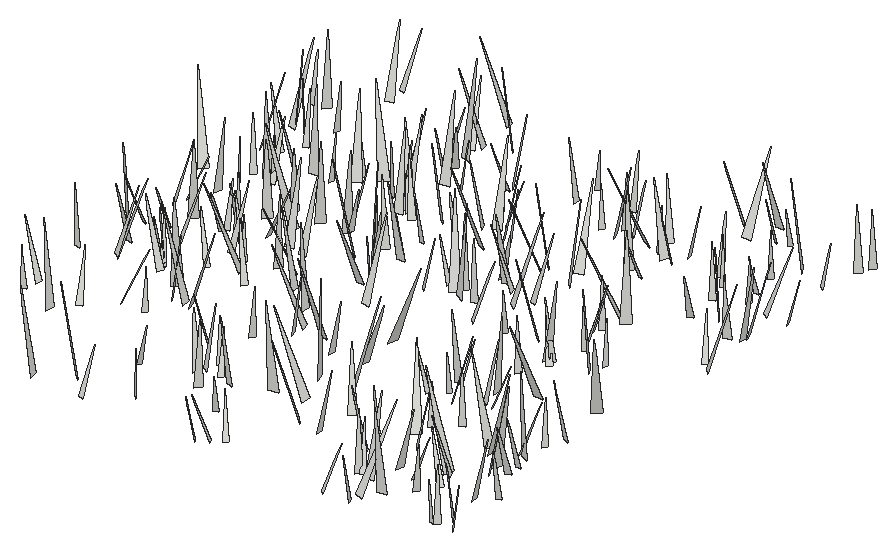
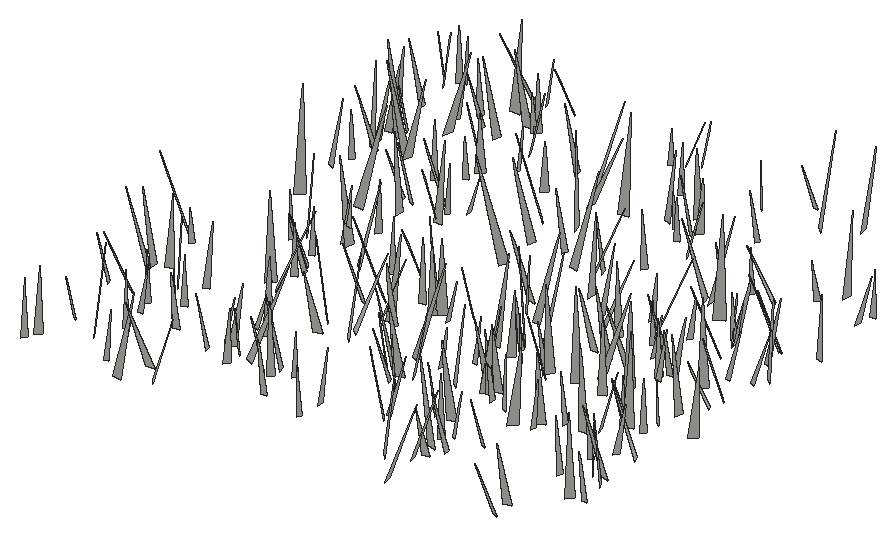
# SketchUp Ruby script. Lengths in inches.
U = 1.inch
M = Sketchup.active_model
def pt(a) = Geom::Point3d.new(a.map { |v| v * U })
def face(e, loops, mat)
  f = e.add_face(loops[0].map { |a| pt(a) })
  loops[1..].each { |l| e.add_face(l.map { |a| pt(a) }).erase! }
  f.material = f.back_material = mat if mat
  f
end
# faces: each face lists its corners as indices into pts; further lists are holes
def faces(e, pts, list, mat = nil) = list.each { |f| face(e, (f[0].is_a?(Array) ? f : [f]).map { |l| l.map { |i| pts[i] } }, mat) }
# xy, xz, yz: faces in a plane at the given z, y or x. An outline is a flat list of corners, or four numbers for a rectangle; further outlines are holes
def ring(l) = l.size == 4 ? [[l[0], l[1]], [l[2], l[1]], [l[2], l[3]], [l[0], l[3]]] : l.each_slice(2).to_a
def flat(e, list, mat, &to3) = list.each { |f| face(e, (f[0].is_a?(Array) ? f : [f]).map { |l| ring(l).map { |u, v| to3.(u, v) } }, mat) }
def xy(e, z, list, mat = nil) = flat(e, list, mat) { |x, y| [x, y, z] }
def xz(e, y, list, mat = nil) = flat(e, list, mat) { |x, z| [x, y, z] }
def yz(e, x, list, mat = nil) = flat(e, list, mat) { |y, z| [x, y, z] }
def lines(e, pts, list) = list.each { |a, b| e.add_line(pt(pts[a]), pt(pts[b])) }
# prism: a flat outline (further loops are holes) pulled along v
def prism(e, loops, v, mat = nil)
  f = face(e, loops, mat); d = Geom::Vector3d.new(v.map { |x| x * U })
  f.pushpull(f.normal.samedirection?(d) ? d.length : -d.length)
end
def box(e, o, s, mat = nil) = prism(e, [[o, [o[0] + s[0], o[1], o[2]], [o[0] + s[0], o[1] + s[1], o[2]], [o[0], o[1] + s[1], o[2]]]], [0, 0, s[2]], mat)
def at(x, y, z, deg = 0) = Geom::Transformation.translation(pt([x, y, z])) * Geom::Transformation.rotation(ORIGIN, Z_AXIS, deg.degrees)
def axes(o, x, y, z) = Geom::Transformation.new([*x, 0, *y, 0, *z, 0, *pt(o).to_a, 1])
def part(name) = M.definitions.add(name)
# library, detail: a bought-in or finely detailed component or shape, given as its bounding box
def library(name, o, s) = part(name).tap { |d| box(d.entities, o, s) }
def detail(e, o, s) = box(e.add_group.entities, o, s)
def put(e, d, t, mat = nil) = e.add_instance(d, t).tap { |i| i.material = mat if mat }
def group(e, t, mat = nil) = e.add_group.tap { |g| g.transformation = t; g.material = mat if mat }.entities
root = M.entities
c1 = part("fur_instance\#9")
p = [[0.8125,0,1.79],[0.67,-0.02,1.48],[0,-0.11,0],[0,0.11,0]]
faces(c1.entities,p,[[0,1,2,3]])
put(root,c1,axes([503.7,262.17,-21.66],[2.36967,1.89121,2.13493],[2.35412,-2.86396,-0.07595],[-1.61018,-1.40392,3.03088]))
put(root,c1,axes([532.14,262.03,-21.66],[-3.28529,-1.60429,1.12724],[-1.66632,3.44368,0.04462],[1.03333,0.45264,3.6558]))
put(root,c1,axes([473.92,262.57,-21.66],[-6.8866,-1.44069,2.04712],[-1.4724,7.17733,0.09795],[2.02444,0.3193,7.035]))
put(root,c1,axes([505.68,263.29,-21.66],[-3.47734,-1.80435,0.22841],[-1.8088,3.48242,-0.02761],[0.19,0.12974,3.9175]))
put(root,c1,axes([527.41,261.63,-21.66],[2.54826,3.20038,0.28055],[3.20908,-2.5526,-0.02947],[-0.15164,-0.23787,4.09087]))
put(root,c1,axes([483.3,261.68,-21.66],[0.89706,4.01856,0.51185],[4.05094,-0.89322,-0.08685],[-0.02607,-0.51851,4.11655]))
put(root,c1,axes([545.09,264.49,-21.66],[-0.48209,-3.49328,1.24378],[-3.69826,0.54426,0.09516],[0.26993,1.21786,3.5251]))
put(root,c1,axes([546.02,264.64,-21.66],[-2.69115,3.5868,1.84623],[3.86426,2.92918,-0.05799],[1.15809,-1.43902,4.48375]))
put(root,c1,axes([548.86,264.65,-21.66],[-2.22453,-2.28888,1.93607],[-2.6411,2.63697,0.08289],[1.41842,1.32035,3.19071]))
put(root,c1,axes([479,266.04,-21.66],[-5.20637,-5.83633,2.28098],[-6.06397,5.44004,0.07832],[1.57922,1.64775,7.82067]))
put(root,c1,axes([507.56,264.51,-21.66],[-2.46678,3.0111,0.36551],[3.02886,2.4705,0.08915],[0.1623,-0.33942,3.8915]))
put(root,c1,axes([534.27,266.7,-21.66],[0.04247,-7.07988,2.41623],[-7.48051,-0.06275,-0.05238],[-0.06984,2.41579,7.07981]))
put(root,c1,axes([489.21,266.67,-21.66],[-2.0645,-2.99831,1.70133],[-3.28642,2.31061,0.08412],[1.04107,1.34824,3.63936]))
put(root,c1,axes([547.11,267.03,-21.66],[-3.81411,-2.18756,1.38745],[-2.30966,3.98998,-0.05835],[1.17299,0.74331,4.39652]))
put(root,c1,axes([532.3125,263.92,-21.66],[2.76635,7.35948,0.05567],[7.35952,-2.76581,-0.07342],[0.04914,-0.07794,7.86188]))
put(root,c1,axes([500.875,270.59,-21.66],[2.15592,-3.18911,0.31319],[-3.19535,-2.16794,-0.07942],[-0.24138,0.21478,3.84865]))
put(root,c1,axes([528.03,269.25,-21.66],[-3.99726,2.72851,1.81883],[2.89094,4.28575,-0.07581],[1.5477,-0.9584,4.83912]))
put(root,c1,axes([537.71,270.27,-21.66],[-2.80028,2.24736,2.49663],[2.73085,3.4158,-0.01176],[1.95607,-1.55147,3.59055]))
put(root,c1,axes([530.31,268.78,-21.66],[0.3651,6.79595,1.75212],[7.01816,-0.34958,-0.10649],[0.01583,-1.75528,6.80491]))
put(root,c1,axes([528.58,269.49,-21.66],[-2.41477,3.3901,0.55663],[3.41153,2.44646,-0.10002],[0.40504,-0.3947,4.161]))
put(root,c1,axes([535.15,272.91,-21.66],[4.26673,-0.51352,0.23406],[-0.5171,-4.27238,0.05285],[-0.22604,0.08052,4.29719]))
put(root,c1,axes([531.66,274.01,-21.66],[5.79925,-1.98106,0.58125],[-1.98372,-5.82701,-0.06806],[-0.57211,0.1232,6.12791]))
put(root,c1,axes([545.76,273.52,-21.66],[5.31059,0.52385,1.16283],[0.52648,-5.43598,0.04446],[-1.16164,-0.06886,5.33618]))
put(root,c1,axes([483.73,274.41,-21.66],[3.66443,-1.25509,0.51627],[-1.25966,-3.69872,-0.05095],[-0.50503,0.11865,3.87307]))
put(root,c1,axes([539.72,273.26,-21.66],[-3.84574,2.31871,0.01808],[2.31862,3.84577,-0.02193],[0.02681,0.00945,4.49062]))
put(root,c1,axes([494.51,274.5,-21.66],[4.30224,-3.16543,2.15858],[-3.43037,-4.62804,0.05027],[-1.70646,1.32286,5.34104]))
put(root,c1,axes([511.87,275.81,-21.66],[-4.79453,-5.10071,1.01007],[-5.15614,4.84133,-0.02673],[0.67211,0.75447,7.00029]))
put(root,c1,axes([524.97,274.87,-21.66],[-4.98874,-1.77944,1.14235],[-1.81158,5.1064,0.04294],[1.09068,0.3424,5.29642]))
put(root,c1,axes([548.35,275.79,-21.66],[1.07632,-4.38935,0.89904],[-4.4763,-1.09335,0.02097],[-0.19334,0.87825,4.51934]))
put(root,c1,axes([516.25,274.92,-21.66],[5.41159,0.09186,1.28906],[0.07062,-5.56242,0.09991],[-1.29039,0.08081,5.41145]))
put(root,c1,axes([538.75,276.86,-21.66],[-4.66141,-1.64687,0.68606],[-1.65466,4.70851,0.06011],[0.66704,0.1713,4.94341]))
put(root,c1,axes([497.46,277.85,-21.66],[-1.75963,-5.21212,1.71135],[-5.46295,1.82898,-0.04671],[0.50104,1.63703,5.50093]))
put(root,c1,axes([537.97,277.33,-21.66],[-8.02945,1.44749,0.94959],[1.4539,8.08421,-0.0293],[0.93976,-0.13944,8.15883]))
put(root,c1,axes([491.58,277.75,-21.66],[-4.02288,2.74208,1.38872],[2.85785,4.17888,0.02734],[1.13147,-0.80565,4.86845]))
put(root,c1,axes([463.69,279.07,-21.66],[-6.94561,0.7265,2.56424],[0.79665,7.39636,0.06233],[2.54332,-0.33278,6.98322]))
put(root,c1,axes([503.6,280.3,-21.66],[1.30407,-7.61557,2.3618],[-7.95747,-1.39423,-0.10194],[-0.50366,2.30972,7.72574]))
put(root,c1,axes([495.13,278.84,-21.66],[-1.61358,3.38665,0.61033],[3.4322,1.63258,0.01498],[0.24881,-0.55751,3.75138]))
put(root,c1,axes([523.21,279.71,-21.66],[-3.75742,-0.36081,1.22113],[-0.40687,3.94545,-0.08619],[1.20657,0.20686,3.77372]))
put(root,c1,axes([492.12,279.05,-21.66],[2.52877,4.50107,1.40807],[4.66336,-2.62485,0.01569],[-0.70386,-1.21962,5.16276]))
put(root,c1,axes([544.91,282.3125,-21.66],[1.17594,-4.92519,0.34785],[-4.93492,-1.18388,-0.07952],[-0.1583,0.31979,5.06301]))
put(root,c1,axes([542.87,280.57,-21.66],[3.30994,1.56111,0.94089],[1.62723,-3.40964,-0.0672],[-0.82125,-0.46405,3.659]))
put(root,c1,axes([529.89,280.22,-21.66],[3.54809,3.00738,1.07129],[3.07779,-3.64774,0.04651],[-0.84804,-0.65624,4.65093]))
put(root,c1,axes([457.1,281.34,-21.66],[1.04159,-3.44564,1.2731],[-3.64709,-1.12789,-0.06873],[-0.4381,1.19732,3.59897]))
put(root,c1,axes([508.86,281.11,-21.66],[-7.40149,0.22253,0.007],[0.22253,7.40149,0.00759],[0.00677,-0.0078,7.40483]))
put(root,c1,axes([492.89,281.5,-21.66],[1.88047,-2.78184,1.95652],[-3.20631,-2.19563,-0.04014],[-1.13412,1.59479,3.35756]))
put(root,c1,axes([542.47,282.83,-21.66],[7.05562,-2.47543,1.6862],[-2.53392,-7.23407,-0.01726],[-1.59697,0.54154,7.47725]))
put(root,c1,axes([516.67,281.93,-21.66],[-3.66348,3.88372,0.60062],[3.90017,3.69385,-0.09601],[0.48235,-0.37054,5.33808]))
put(root,c1,axes([488.92,284.06,-21.66],[-3.66395,-2.75565,0.79106],[-2.79858,3.7164,-0.01609],[0.62239,0.48852,4.58453]))
put(root,c1,axes([544.86,284.65,-21.66],[-0.84306,-4.44176,0.86686],[-4.52258,0.85891,0.00263],[0.16427,0.85115,4.52106]))
put(root,c1,axes([466.31,282.45,-21.66],[-1.50833,4.20798,0.27956],[4.21722,1.50618,0.08227],[0.01672,-0.29093,4.46939]))
put(root,c1,axes([457.63,284.17,-21.66],[-4.98087,1.16288,0.32288],[1.15979,4.99131,-0.08543],[0.33384,0.00996,5.1141]))
put(root,c1,axes([527.28,283.33,-21.66],[-4.42637,5.44798,0.10976],[5.44745,4.42761,-0.08267],[0.13338,-0.03304,7.019]))
put(root,c1,axes([539.19,285.53,-21.66],[7.16515,0.1083,1.44204],[0.09788,-7.3087,0.06254],[-1.44279,0.042,7.1657]))
put(root,c1,axes([527.66,286.15,-21.66],[1.56835,-2.82264,1.69633],[-3.20586,-1.73838,0.07137],[-0.75322,1.52161,3.2283]))
put(root,c1,axes([474.875,286.87,-21.66],[-2.3678,2.48019,1.72309],[2.76192,2.66404,-0.03926],[1.22155,-1.2159,3.42875]))
put(root,c1,axes([537.98,286.61,-21.66],[-7.39383,1.79038,1.19471],[1.82356,7.48136,0.07416],[1.14343,-0.35412,7.60715]))
put(root,c1,axes([543.77,287.375,-21.66],[2.87262,5.81566,3.24646],[6.49078,-3.23727,0.05584],[-1.49368,-2.88298,6.48619]))
put(root,c1,axes([506.33,287.46,-21.66],[7.01213,2.59998,3.36264],[2.81322,-7.70163,0.08845],[-3.18638,-1.07803,7.47811]))
put(root,c1,axes([470.45,287.08,-21.66],[4.47916,2.33614,0.04477],[2.33654,-4.47877,-0.05982],[-0.01203,-0.07375,5.05142]))
put(root,c1,axes([542.66,287.96,-21.66],[5.19271,0.37939,0.34653],[0.38191,-5.20401,-0.02543],[-0.34375,-0.05067,5.20649]))
put(root,c1,axes([530.99,289.25,-21.66],[1.68942,-4.24341,1.91691],[-4.60334,-1.82876,0.00876],[-0.70022,1.78447,4.56734]))
put(root,c1,axes([511.6,288.69,-21.66],[5.53821,4.98185,1.27941],[5.04776,-5.62536,0.05401],[-0.98782,-0.81487,7.449]))
put(root,c1,axes([491.43,290.72,-21.66],[3.58428,-2.61771,1.24135],[-2.70899,-3.7283,-0.04015],[-1.02701,0.69843,4.43823]))
put(root,c1,axes([544.11,291.72,-21.66],[-2.72992,2.63061,1.69887],[2.87463,2.99911,-0.02472],[1.24209,-1.1593,3.79104]))
put(root,c1,axes([477.83,292.48,-21.66],[-7.83982,-0.95667,1.33619],[-0.96404,7.9519,0.03699],[1.33088,0.12461,7.89789]))
put(root,c1,axes([475.53,292.26,-21.66],[4.582,2.26461,1.64468],[2.3704,-4.81752,0.02956],[-1.48816,-0.70087,5.111]))
put(root,c1,axes([478.9,292.19,-21.66],[6.34041,1.92452,0.88463],[1.94009,-6.39712,0.01179],[-0.84995,-0.24555,6.62604]))
put(root,c1,axes([521.17,293.61,-21.66],[-3.91396,0.19988,0.40503],[0.19284,3.93443,-0.07818],[0.40843,0.05784,3.91828]))
put(root,c1,axes([503.17,294.04,-21.66],[4.73571,-1.08461,0.9225],[-1.0987,-4.82145,-0.02851],[-0.90568,0.17765,4.85824]))
put(root,c1,axes([508.71,294.81,-21.66],[6.16535,-1.94029,0.16764],[-1.94054,-6.16752,-0.01601],[-0.16472,0.03505,6.46343]))
put(root,c1,axes([545.17,295.05,-21.66],[-1.95958,-4.83915,1.26512],[-4.97855,2.01787,0.00704],[0.48156,1.1699,5.22085]))
put(root,c1,axes([473.6875,295.65,-21.66],[3.80262,-6.94068,2.14426],[-7.19034,-3.9408,-0.00453],[-1.0344,1.87826,7.9141]))
put(root,c1,axes([525.47,293.91,-21.66],[4.69542,3.0157,0.91715],[3.05189,-4.76105,0.03053],[-0.78841,-0.46959,5.58037]))
put(root,c1,axes([499.41,296.93,-21.66],[-2.16653,-7.31637,0.90738],[-7.36569,2.18851,0.05952],[0.3151,0.85299,7.63018]))
put(root,c1,axes([523.5,295.61,-21.66],[1.81522,-3.21568,0.8696],[-3.29805,-1.87418,-0.04607],[-0.46866,0.73395,3.69235]))
put(root,c1,axes([495.33,295.16,-21.66],[4.4988,1.24272,1.44893],[1.33102,-4.70119,-0.10058],[-1.36826,-0.48722,4.6662]))
put(root,c1,axes([455.36,295.72,-21.66],[1.09401,4.63876,2.44173],[5.21296,-1.22556,-0.00737],[-0.55243,-2.37843,4.76601]))
put(root,c1,axes([531.0625,296.09,-21.66],[3.86213,1.08614,0.2172],[1.09096,-3.86634,-0.0646],[-0.19154,-0.12107,4.01143]))
put(root,c1,axes([495.47,297.57,-21.66],[-6.50715,-2.26194,0.29712],[-2.26712,6.51165,-0.07913],[0.25462,0.17236,6.88863]))
put(root,c1,axes([529.4375,296.45,-21.66],[2.64561,4.33348,1.24236],[4.47199,-2.70465,-0.08904],[-0.56902,-1.10798,5.07645]))
put(root,c1,axes([522.83,298.63,-21.66],[0.27233,-6.25887,1.87066],[-6.53155,-0.29195,-0.02597],[-0.1084,1.8677,6.26474]))
put(root,c1,axes([469.08,297.55,-21.66],[-5.48361,2.04542,0.49712],[2.0602,5.49974,0.09665],[0.43181,-0.2646,5.85187]))
put(root,c1,axes([524,297.5625,-21.66],[2.95956,2.83712,0.75066],[2.89518,-2.997,-0.08741],[-0.48027,-0.58351,4.09885]))
put(root,c1,axes([461.68,297.09,-21.66],[4.96936,4.425,0.65774],[4.44372,-4.99597,0.03757],[-0.51632,-0.4092,6.65385]))
put(root,c1,axes([461.31,297.24,-21.66],[3.13584,4.70476,0.63652],[4.72939,-3.16238,0.0748],[-0.41563,-0.48786,5.65355]))
put(root,c1,axes([534.39,302.33,-21.66],[-0.28609,-7.90952,0.17476],[-7.91116,0.28452,-0.07401],[-0.06767,0.17732,7.91434]))
put(root,c1,axes([468.52,298.81,-21.66],[-1.71851,4.03919,1.0736],[4.16688,1.74577,0.10182],[0.32374,-1.02868,4.3884]))
put(root,c1,axes([467.48,299.8,-21.66],[-3.40834,-0.81843,0.94444],[-0.85751,3.5273,-0.03792],[0.90911,0.25869,3.50503]))
put(root,c1,axes([528.77,299.88,-21.66],[6.1687,-0.67373,2.21616],[-0.70194,-6.55164,-0.0379],[-2.20738,0.2006,6.20527]))
put(root,c1,axes([467.7,300.24,-21.66],[-3.21218,-2.63282,1.4726],[-2.81239,3.39173,-0.07071],[1.09119,0.99138,4.15269]))
put(root,c1,axes([460.17,301.5625,-21.66],[-1.26664,-5.03308,1.07763],[-5.14261,1.28411,-0.04714],[0.2163,1.05675,5.1898]))
put(root,c1,axes([507.95,302.06,-21.66],[8.10386,-2.02713,0.06413],[-2.02706,-8.10412,-0.01624],[-0.06615,-0.00019,8.35354]))
put(root,c1,axes([492.31,301.76,-21.66],[-6.58404,0.20466,2.39247],[0.20033,7.00521,-0.04793],[2.39284,-0.02336,6.58705]))
put(root,c1,axes([543.59,304.23,-21.66],[4.25947,-6.86655,0.67935],[-6.89421,-4.26807,0.08653],[-0.2843,0.62304,8.07992]))
put(root,c1,axes([481,301.82,-21.66],[-3.95377,2.90545,0.68572],[2.92437,3.99824,-0.07937],[0.59996,-0.34142,4.90588]))
put(root,c1,axes([473.61,302.51,-21.66],[-3.58743,2.64736,0.43412],[2.66538,3.59954,0.07504],[0.30449,-0.3184,4.45786]))
put(root,c1,axes([477.97,304.68,-21.66],[-6.75441,-2.93713,0.31923],[-2.94167,6.75982,-0.04619],[0.27431,0.1697,7.36523]))
put(root,c1,axes([457.1875,305.06,-21.66],[-4.34525,-4.69158,2.51984],[-5.05188,4.66036,-0.03462],[1.68493,1.87398,6.3946]))
put(root,c1,axes([487.51,305.26,-21.66],[-6.3571,-0.05635,1.63328],[-0.03082,6.56286,0.10646],[1.63396,-0.09544,6.35645]))
put(root,c1,axes([467.11,303.86,-21.66],[4.12664,4.96749,0.53315],[4.97839,-4.14664,0.10195],[-0.41933,-0.34468,6.45715]))
put(root,c1,axes([458.4375,307.16,-21.66],[-1.93771,-4.14246,0.35212],[-4.15628,1.93921,-0.05843],[0.0961,0.34375,4.57288]))
put(root,c1,axes([527.59,306.21,-21.66],[3.42061,-2.16163,2.16053],[-2.46149,-3.8706,0.02453],[-1.81151,1.17767,4.04631]))
put(root,c1,axes([461.96,308.34,-21.66],[-0.71572,-3.67555,0.46048],[-3.70429,0.70984,-0.09154],[-0.00255,0.46948,3.74347]))
put(root,c1,axes([476.59,307.19,-21.66],[-1.48065,3.15767,1.46809],[3.42197,1.61497,-0.02236],[0.64523,-1.31889,3.48751]))
put(root,c1,axes([484.46,309.35,-21.66],[-3.64802,-5.0358,0.07825],[-5.03596,3.64854,0.02575],[0.06676,0.04827,6.21825]))
put(root,c1,axes([481.78,308.7,-21.66],[5.0258,-2.8928,2.35137],[-3.11716,-5.42578,-0.01254],[-2.04464,1.16127,5.79886]))
put(root,c1,axes([473.82,307.8125,-21.66],[1.01663,5.56132,0.68679],[5.60282,-1.02017,-0.03274],[-0.09106,-0.68151,5.65338]))
put(root,c1,axes([493.64,312.56,-21.66],[-0.44109,-6.89492,0.21564],[-6.89758,0.44393,0.08524],[0.09888,0.20974,6.90849]))
put(root,c1,axes([498.125,308.09,-21.66],[1.00933,7.00307,0.82634],[7.04916,-1.02422,0.06983],[-0.18746,-0.80782,7.07509]))
put(root,c1,axes([468.7,312.03,-21.66],[0.77798,-4.23548,0.16889],[-4.23878,-0.77834,0.00619],[-0.02442,0.16723,4.30633]))
put(root,c1,axes([474.21,309.91,-21.66],[-3.97928,1.73175,0.54979],[1.73454,4.01483,-0.09183],[0.54094,-0.13447,4.3388]))
put(root,c1,axes([496.54,311.3,-21.66],[-3.07228,-3.20464,1.70758],[-3.41257,3.31254,0.07678],[1.24093,1.17551,4.43878]))
put(root,c1,axes([528.55,311.61,-21.66],[6.63487,-1.65212,1.91106],[-1.73662,-6.8834,0.0785],[-1.83462,0.54083,6.83702]))
put(root,c1,axes([529.74,311.5,-21.66],[-4.97089,0.8761,1.32855],[0.91857,5.13772,0.0489],[1.29955,-0.28038,5.04727]))
put(root,c1,axes([463.19,312.5,-21.66],[4.72126,-4.87179,1.88096],[-5.03873,-4.91595,-0.08523],[-1.37242,1.28908,6.78361]))
put(root,c1,axes([529.72,310.73,-21.66],[-3.26703,2.9675,0.38966],[2.97957,3.27925,0.00816],[0.28293,-0.26806,4.41355]))
put(root,c1,axes([535.25,312.92,-21.66],[-5.46396,-3.21591,2.3792],[-3.43589,5.83542,-0.00311],[2.04873,1.20967,6.3401]))
put(root,c1,axes([469.13,312.71,-21.66],[-0.34348,3.88251,1.09091],[4.02925,0.37671,-0.07204],[0.17064,-1.07988,3.89701]))
put(root,c1,axes([518.67,314.28,-21.66],[2.48728,-3.44318,0.65298],[-3.47724,-2.52444,-0.0662],[-0.43662,0.49004,4.24707]))
put(root,c1,axes([470.12,313.97,-21.66],[3.33409,-2.8819,1.80128],[-3.12207,-3.59416,0.02846],[-1.34262,1.20116,4.40689]))
put(root,c1,axes([469.6,314.71,-21.66],[-0.47471,-3.8388,0.84095],[-3.92781,0.49062,0.02236],[0.12592,0.83177,3.86797]))
put(root,c1,axes([523.57,315.71,-21.66],[-4.39451,-5.32367,1.29551],[-5.40377,4.48556,0.10243],[0.905,0.93264,6.90237]))
put(root,c1,axes([458.69,313.61,-21.66],[3.76051,3.97563,0.83952],[4.01253,-3.81366,0.08642],[-0.64034,-0.54974,5.47171]))
put(root,c1,axes([513.06,313.82,-21.66],[3.32598,3.77438,0.4675],[3.78797,-3.34308,0.04133],[-0.34022,-0.32329,5.03054]))
put(root,c1,axes([474.84,315.13,-21.66],[4.99939,-0.31235,0.02616],[-0.31267,-4.999,0.06629],[-0.02197,0.06779,5.0087]))
put(root,c1,axes([536.15,315.38,-21.66],[-3.33469,1.40616,1.82105],[1.56398,3.73727,-0.02186],[1.68745,-0.685,3.61897]))
put(root,c1,axes([482.02,313.85,-21.66],[0.04484,6.03011,0.93276],[6.10111,-0.02998,-0.09948],[0.09373,-0.93336,6.02946]))
put(root,c1,axes([479.26,314.38,-21.66],[-0.62472,6.74476,1.37593],[6.88336,0.62526,0.06028],[0.06565,-1.37569,6.77336]))
put(root,c1,axes([531,317.12,-21.66],[1.90593,-3.10212,1.28599],[-3.27722,-2.04084,-0.06594],[-0.73267,1.05893,3.64024]))
put(root,c1,axes([458.91,316.5,-21.66],[3.47844,1.93474,0.04271],[1.93521,-3.47755,-0.07868],[0.00093,-0.08952,3.97952]))
put(root,c1,axes([487.76,318.45,-21.66],[4.25123,5.18566,4.75994],[6.35301,-5.22113,0.01405],[-3.03108,-3.67013,6.70551]))
put(root,c1,axes([501.71,316.91,-21.66],[3.13745,2.7412,0.96065],[2.81213,-3.22064,0.00574],[-0.7273,-0.62763,4.16626]))
put(root,c1,axes([509.96,318.3,-21.66],[-0.91503,4.79321,2.31879],[5.31141,0.98733,0.05504],[0.37492,-2.28894,4.87946]))
put(root,c1,axes([507.33,318.08,-21.66],[3.62939,6.32437,2.66269],[6.74766,-3.83695,-0.08396],[-1.24771,-2.35377,7.2913]))
put(root,c1,axes([471.43,319.08,-21.66],[4.24659,-4.94069,2.32668],[-5.22174,-4.53655,-0.10277],[-1.59916,1.69313,6.51409]))
put(root,c1,axes([491.06,318.51,-21.66],[5.9616,4.7587,3.0284],[5.08757,-6.43918,0.10304],[-2.43578,-1.80245,7.62727]))
put(root,c1,axes([476.54,318.82,-21.66],[-8.26176,0.40654,0.83522],[0.41692,8.30295,0.08258],[0.83009,-0.12394,8.27135]))
put(root,c1,axes([490.36,320.05,-21.66],[3.76138,-1.24538,0.93866],[-1.27843,-3.86595,-0.00634],[-0.89313,0.28885,3.96218]))
put(root,c1,axes([493.94,321.43,-21.66],[-0.46017,-7.01963,1.64197],[-7.20868,0.46604,-0.02793],[0.07879,1.64032,7.03464]))
put(root,c1,axes([503.76,320.09,-21.66],[-3.79892,0.58903,0.61511],[0.5899,3.84804,-0.04166],[0.61427,-0.05255,3.84409]))
put(root,c1,axes([506.5,320.26,-21.66],[-5.0872,2.66073,2.45988],[2.85923,5.55214,-0.09239],[2.22604,-1.05084,5.74025]))
put(root,c1,axes([505.71,319.05,-21.66],[-4.53452,6.13099,1.20513],[6.2123,4.58336,0.05748],[0.66981,-1.00349,7.62546]))
put(root,c1,axes([460.99,320.78,-21.66],[5.93404,-1.49093,1.99542],[-1.59561,-6.23409,0.08712],[-1.91274,0.57506,6.11785]))
put(root,c1,axes([529.53,319.93,-21.66],[3.18185,3.17768,0.5905],[3.1987,-3.21478,0.06397],[-0.46337,-0.37158,4.49642]))
put(root,c1,axes([478.29,322.61,-21.66],[5.05478,-5.09898,2.04992],[-5.28407,-5.27475,-0.09077],[-1.51011,1.38923,7.17929]))
put(root,c1,axes([528.55,321.91,-21.66],[4.6292,0.17151,0.50537],[0.17521,-4.6565,-0.02456],[-0.5041,-0.0434,4.63231]))
put(root,c1,axes([493.68,322.36,-21.66],[-3.08604,-1.58363,1.00431],[-1.62158,3.22493,0.10239],[0.94181,0.36349,3.46714]))
put(root,c1,axes([473.125,323.16,-21.66],[3.25628,-4.96201,1.27437],[-5.08219,-3.31911,0.06246],[-0.64574,1.10043,5.93473]))
put(root,c1,axes([482.875,322.875,-21.66],[-5.61419,2.77509,3.47904],[3.15086,6.4338,-0.04739],[3.14276,-1.49299,6.26243]))
put(root,c1,axes([490.25,322.42,-21.66],[-4.38445,3.57185,1.79964],[3.76738,4.58485,0.07863],[1.34299,-1.20052,5.65467]))
put(root,c1,axes([514.83,320.9,-21.66],[4.48947,6.23838,0.89691],[6.27438,-4.52789,0.08708],[-0.59503,-0.67674,7.68539]))
put(root,c1,axes([488.24,322.85,-21.66],[2.1369,3.02619,1.55246],[3.28055,-2.31782,0.00255],[-0.89775,-1.26656,3.70461]))
put(root,c1,axes([483.18,323.45,-21.66],[3.78435,-1.32179,0.68035],[-1.35222,-3.83372,0.07338],[-0.61764,0.29457,4.00787]))
put(root,c1,axes([529.15,323.47,-21.66],[1.67153,-3.68103,1.97281],[-4.08391,-1.88531,-0.05752],[-0.87388,1.76964,4.04237]))
put(root,c1,axes([512.12,324.19,-21.66],[-5.21279,-1.15752,0.50027],[-1.17064,5.23306,-0.0898],[0.46875,0.19648,5.33901]))
put(root,c1,axes([510.08,325.45,-21.66],[1.37866,-6.43403,1.32521],[-6.55871,-1.42426,-0.09169],[-0.36909,1.27608,6.57944]))
put(root,c1,axes([461.67,324.82,-21.66],[1.95949,2.80373,1.45551],[3.04239,-2.136,0.01872],[-0.85045,-1.18135,3.42055]))
put(root,c1,axes([516.52,323.42,-21.66],[2.68207,4.86571,0.6841],[4.89534,-2.71316,0.10499],[-0.42283,-0.54794,5.55496]))
put(root,c1,axes([548.44,323.49,-21.66],[5.3088,5.05785,1.00754],[5.10033,-5.36326,0.04959],[-0.76398,-0.65873,7.33231]))
put(root,c1,axes([482.64,324.35,-21.66],[3.62084,3.81527,1.03017],[3.87963,-3.69771,0.05854],[-0.75237,-0.70613,5.25959]))
put(root,c1,axes([508.8125,326.06,-21.66],[3.98619,-2.41358,0.43201],[-2.42835,-4.00018,0.05811],[-0.33929,0.27366,4.65958]))
put(root,c1,axes([546.71,325.02,-21.66],[-2.11834,3.44874,0.2067],[3.45458,2.11778,0.0692],[0.04913,-0.21236,4.04678]))
put(root,c1,axes([455.26,324.63,-21.66],[-5.44191,5.3364,0.6963],[5.36336,5.45938,0.07682],[0.44311,-0.54257,7.6214]))
put(root,c1,axes([528.84,328.02,-21.66],[-5.75391,-4.14909,0.07824],[-4.14913,5.75437,0.02082],[0.07564,0.02888,7.0938]))
put(root,c1,axes([493.09,327.31,-21.66],[-1.22069,-3.41408,1.05948],[-3.55821,1.26785,-0.01408],[0.34288,1.00256,3.62571]))
put(root,c1,axes([530.64,327.08,-21.66],[5.17413,-4.7343,3.23528],[-5.24163,-5.67192,0.08293],[-2.32507,2.25121,7.01272]))
put(root,c1,axes([464.33,328.22,-21.66],[2.05152,-6.96349,2.48946],[-7.36809,-2.14532,0.07104],[-0.63146,2.40909,7.25905]))
put(root,c1,axes([465.36,328.16,-21.66],[2.21811,-2.97156,1.30139],[-3.14682,-2.35396,-0.01147],[-0.78819,1.03561,3.7081]))
put(root,c1,axes([461.8,327.96,-21.66],[2.76185,-3.07557,2.49035],[-3.57907,-3.23702,-0.02845],[-1.68858,1.83068,4.13354]))
put(root,c1,axes([512.22,330.87,-21.66],[-4.64993,-4.92524,0.42817],[-4.93518,4.6591,-0.00251],[0.29211,0.31306,6.77347]))
put(root,c1,axes([465.56,327.26,-21.66],[-0.62554,4.99616,0.12365],[4.99768,0.62512,0.02455],[-0.009,-0.12574,5.03511]))
put(root,c1,axes([500.61,331.52,-21.66],[-3.23676,-6.95107,0.75182],[-6.9834,3.25434,0.02332],[0.33861,0.67166,7.66769]))
put(root,c1,axes([466.89,331.43,-21.66],[-4.90354,-1.85753,0.89414],[-1.8937,4.97041,-0.05944],[0.81474,0.37312,5.24324]))
put(root,c1,axes([517.3,330.69,-21.66],[-4.33935,-4.28478,3.74469],[-5.00881,5.11096,0.04388],[2.70071,2.59437,6.09815]))
put(root,c1,axes([496.04,331.28,-21.66],[-3.46887,0.5768,0.94943],[0.60796,3.5911,0.03958],[0.92978,-0.19616,3.51628]))
put(root,c1,axes([544.63,332.74,-21.66],[1.69924,-5.28596,1.58911],[-5.50046,-1.7602,0.02657],[-0.46001,1.5213,5.5523]))
put(root,c1,axes([511.7,332.96,-21.66],[-4.72321,-4.87597,2.05821],[-5.0831,4.94763,0.05633],[1.47426,1.43735,6.78828]))
put(root,c1,axes([536.71,334.16,-21.66],[2.00782,-4.43373,0.05819],[-4.43409,-2.00742,0.0429],[0.01508,0.0707,4.86698]))
put(root,c1,axes([487.84,331.57,-21.66],[-3.61656,3.24074,0.55892],[3.26072,3.64166,-0.01623],[0.42715,-0.36083,4.85609]))
put(root,c1,axes([471.99,333.07,-21.66],[-3.43259,1.11019,2.13702],[1.24058,4.00441,-0.08763],[2.06406,-0.56053,3.60659]))
put(root,c1,axes([485.18,331.88,-21.66],[-1.64071,6.20292,1.41522],[6.35653,1.66047,0.09149],[0.27128,-1.39198,6.41559]))
put(root,c1,axes([468.6,333.21,-21.66],[-0.16128,6.84934,2.86842],[7.42417,0.20732,-0.07764],[0.15166,-2.86546,6.8508]))
put(root,c1,axes([491.39,334.03,-21.66],[-4.35453,-4.53446,2.05004],[-4.74623,4.60317,0.10013],[1.49574,1.4055,6.28595]))
put(root,c1,axes([546.7,333.73,-21.66],[6.13024,0.22864,1.74835],[0.20896,-6.37456,0.10097],[-1.75081,0.03976,6.13367]))
put(root,c1,axes([484.33,334.28,-21.66],[5.43956,-0.0104,1.6458],[0.01524,-5.68242,-0.08629],[-1.64576,-0.087,5.43889]))
put(root,c1,axes([486.57,332.97,-21.66],[-5.17368,4.83178,0.63052],[4.85594,5.1888,0.08232],[0.40437,-0.49072,7.07858]))
put(root,c1,axes([485.625,333.13,-21.66],[0.08321,7.29137,1.2347],[7.39423,-0.10178,0.10277],[-0.11831,-1.23331,7.29112]))
put(root,c1,axes([481.32,335.19,-21.66],[-1.7362,-3.80786,1.79903],[-4.13168,1.91701,0.07019],[0.81577,1.60498,4.18441]))
put(root,c1,axes([546.71,334.92,-21.66],[6.30339,2.19635,1.13005],[2.22882,-6.39265,-0.00763],[-1.06457,-0.37914,6.67507]))
put(root,c1,axes([457.78,334.71,-21.66],[5.69643,3.12279,1.00252],[3.16084,-5.76326,-0.00802],[-0.87518,-0.48903,6.49623]))
put(root,c1,axes([497.28,336.01,-21.66],[-4.91949,-2.25789,1.34677],[-2.33985,5.06309,-0.05864],[1.19873,0.61667,5.41258]))
put(root,c1,axes([502.79,335.45,-21.66],[3.09566,2.75124,1.27433],[2.88928,-3.22895,-0.04754],[-0.91941,-0.88367,4.14127]))
put(root,c1,axes([501.86,335.17,-21.66],[5.547,2.87669,1.51326],[2.93945,-5.71712,0.09337],[-1.38744,-0.61131,6.24786]))
put(root,c1,axes([460.85,335.24,-21.66],[-4.64621,2.31988,0.55706],[2.32982,4.67441,-0.03457],[0.51391,-0.21773,5.19306]))
put(root,c1,axes([540.16,336.31,-21.66],[-4.40906,-3.22075,2.19411],[-3.50304,4.72714,-0.10035],[1.70765,1.38134,5.45921]))
put(root,c1,axes([474.79,335.25,-21.66],[-3.82919,5.78151,1.38736],[5.88668,3.91838,-0.08139],[0.83523,-1.11076,6.93412]))
put(root,c1,axes([516.27,334.33,-21.66],[-1.83957,6.80237,0.25254],[6.80704,1.83779,0.08208],[-0.01336,-0.2652,7.04624]))
put(root,c1,axes([474.77,336.81,-21.66],[-3.91308,1.33626,1.31278],[1.41439,4.10109,0.04154],[1.2282,-0.46546,4.13474]))
put(root,c1,axes([523.81,338.8,-21.66],[-1.2303,-3.6424,0.32202],[-3.65502,1.23499,0.00478],[0.10759,0.30356,3.84457]))
put(root,c1,axes([499.16,336.9,-21.66],[-1.91608,6.79372,1.10059],[6.8739,1.94553,-0.04218],[0.33984,-1.04766,7.05863]))
put(root,c1,axes([477.66,337.875,-21.66],[-6.04844,4.67756,1.28768],[4.75602,6.12308,0.0974],[0.95811,-0.86582,7.6455]))
put(root,c1,axes([499.44,338.8,-21.66],[4.10602,0.97464,0.35289],[0.9844,-4.11806,-0.08026],[-0.32469,-0.15985,4.21935]))
put(root,c1,axes([462.84,338.59,-21.66],[-1.62337,4.08317,1.17277],[4.21606,1.70273,-0.09236],[0.52201,-1.05424,4.39307]))
put(root,c1,axes([521.2,339.48,-21.66],[4.8811,-3.48072,2.77846],[-3.79933,-5.40519,-0.09683],[-2.32386,1.52607,5.99426]))
put(root,c1,axes([497.99,339.61,-21.66],[3.13012,3.09581,1.75638],[3.35561,-3.34662,-0.08138],[-1.18695,-1.29717,4.40172]))
put(root,c1,axes([535.99,340.12,-21.66],[-2.40866,3.6867,1.3913],[3.88066,2.50239,0.08743],[0.68406,-1.21467,4.40293]))
put(root,c1,axes([548.74,341.34,-21.66],[3.66327,1.41122,0.72087],[1.44956,-3.71776,-0.08822],[-0.64027,-0.34277,3.92471]))
put(root,c1,axes([459.59,342.25,-21.66],[3.22406,2.21993,1.84513],[2.48282,-3.54361,-0.0749],[-1.47248,-1.11442,3.91371]))
put(root,c1,axes([540.6,342.68,-21.66],[2.98723,-2.64764,1.00912],[-2.72025,-3.09017,-0.05514],[-0.79284,0.62671,3.99131]))
put(root,c1,axes([488.04,342.48,-21.66],[3.88099,1.49769,1.22771],[1.56049,-4.04689,0.00388],[-1.14683,-0.43823,4.15995]))
put(root,c1,axes([544.7,341.39,-21.66],[3.10305,4.72146,0.30771],[4.72969,-3.10544,-0.04628],[-0.13026,-0.28259,5.64969]))
put(root,c1,axes([485.26,342.33,-21.66],[-1.01475,7.09695,1.79918],[7.31311,1.06925,-0.09303],[0.3496,-1.76734,7.16853]))
put(root,c1,axes([457.64,341.88,-21.66],[1.8777,6.7714,0.98346],[6.8334,-1.90815,0.09124],[-0.35155,-0.923,7.02632]))
put(root,c1,axes([457.04,343.77,-21.66],[-4.37143,-2.8181,2.86453],[-3.24687,4.97094,-0.06453],[2.3675,1.61389,5.20067]))
put(root,c1,axes([518.65,346.9,-21.66],[-3.40543,-6.99905,0.02732],[-6.9991,3.40539,-0.01642],[-0.00281,0.03175,7.78353]))
put(root,c1,axes([534.7,343.96,-21.66],[-0.32853,3.96848,1.56907],[4.26678,0.33258,0.05223],[0.07349,-1.56822,3.98171]))
put(root,c1,axes([524.65,344.83,-21.66],[-2.53419,-2.69204,0.92744],[-2.77792,2.61003,-0.01451],[0.6248,0.68554,3.69715]))
put(root,c1,axes([539.68,345.52,-21.66],[0.38747,-3.62863,0.53891],[-3.66751,-0.39531,-0.02484],[-0.08219,0.53319,3.64917]))
put(root,c1,axes([463.42,344.93,-21.66],[4.19942,-1.36084,1.21546],[-1.38514,-4.36301,-0.09922],[-1.1877,0.2767,4.41329]))
put(root,c1,axes([493.17,346.79,-21.66],[-1.39577,-4.42794,0.41329],[-4.44248,1.40819,0.08395],[0.20461,0.36877,4.64196]))
put(root,c1,axes([481.99,346.02,-21.66],[-1.43466,-3.23484,0.82707],[-3.31328,1.49057,0.08262],[0.41278,0.72144,3.53774]))
put(root,c1,axes([523.16,345.11,-21.66],[-5.60882,2.54428,1.1021],[2.59069,5.69507,0.03704],[0.9881,-0.48955,6.15881]))
put(root,c1,axes([483.17,347.32,-21.66],[3.21105,-3.45107,0.18225],[-3.45172,-3.21492,-0.06213],[-0.16965,0.09106,4.71348]))
put(root,c1,axes([477.17,345.27,-21.66],[1.79566,3.71313,0.76849],[3.77743,-1.82574,-0.00496],[-0.33004,-0.69403,4.12452]))
put(root,c1,axes([513.52,346.01,-21.66],[5.7925,1.49056,1.34896],[1.52882,-5.93778,-0.00376],[-1.30544,-0.3399,5.9812]))
put(root,c1,axes([510.75,346.42,-21.66],[-2.66914,2.15187,1.53787],[2.38339,2.90414,0.07299],[1.14676,-1.02728,3.42776]))
put(root,c1,axes([521.08,346.1875,-21.66],[-2.34168,-2.41248,1.9117],[-2.76899,2.70012,0.01564],[1.3444,1.35921,3.36204]))
put(root,c1,axes([532.76,345.9375,-21.66],[-0.41482,4.98169,1.32883],[5.15587,0.40286,0.09923],[0.00793,-1.33251,4.99795]))
put(root,c1,axes([513.65,348.22,-21.66],[4.04014,-3.74392,1.13553],[-3.80741,-4.13804,-0.09691],[-0.90002,0.69913,5.50729]))
put(root,c1,axes([525.59,347.8125,-21.66],[4.33952,0.70183,1.00017],[0.70812,-4.45199,0.05164],[-0.99573,-0.10739,4.3956]))
put(root,c1,axes([515.52,347.6875,-21.66],[2.94995,3.39967,1.09614],[3.50655,-3.02709,-0.04841],[-0.68072,-0.86052,4.50085]))
put(root,c1,axes([493.18,348,-21.66],[-3.61899,-3.55384,3.43713],[-4.24844,4.41399,0.09065],[2.52873,2.32973,5.07136]))
put(root,c1,axes([458.0625,349.35,-21.66],[-4.38219,4.14776,3.28171],[4.71988,4.98997,-0.0042],[2.38668,-2.25242,6.03386]))
put(root,c1,axes([455.79,348.88,-21.66],[0.08928,4.21713,1.27448],[4.4055,-0.088,-0.01741],[-0.00879,-1.27457,4.21804]))
put(root,c1,axes([538.54,350.27,-21.66],[2.93376,-3.22318,1.07266],[-3.3076,-3.03341,-0.06853],[-0.77414,0.74566,4.35788]))
put(root,c1,axes([480.125,349.86,-21.66],[4.64255,0.07182,0.51653],[0.0806,-4.67045,-0.07504],[-0.51523,-0.08349,4.6425]))
put(root,c1,axes([520.78,349.29,-21.66],[-3.74669,3.50171,1.17991],[3.59906,3.83892,0.03541],[0.8372,-0.8322,5.12819]))
put(root,c1,axes([502.92,350.33,-21.66],[-4.88413,-0.13594,1.40409],[-0.16648,5.08029,-0.08723],[1.4008,0.12978,4.88524]))
put(root,c1,axes([482.7,350.21,-21.66],[2.51079,7.35519,2.45383],[7.71335,-2.63218,-0.00261],[-0.79014,-2.32314,7.77193]))
put(root,c1,axes([546.01,352.59,-21.66],[1.71748,3.11444,0.84575],[3.20742,-1.75327,-0.057],[-0.35706,-0.7688,3.55615]))
put(root,c1,axes([511.01,353.16,-21.66],[0.37459,4.6587,1.44665],[4.87681,-0.39143,-0.00226],[-0.11359,-1.44218,4.67373]))
put(root,c1,axes([482.69,354.4375,-21.66],[-6.22564,-1.43503,0.72375],[-1.44178,6.26598,0.02194],[0.71021,0.14105,6.38885]))
put(root,c1,axes([540.74,354.75,-21.66],[-6.29622,-3.82649,2.40942],[-4.00808,6.63484,0.06324],[2.09347,1.19444,7.36752]))
put(root,c1,axes([503.11,354.92,-21.66],[2.68413,-2.59886,0.79499],[-2.66781,-2.73276,0.07385],[-0.51851,0.60713,3.7354]))
put(root,c1,axes([481.82,352.6875,-21.66],[-1.75814,5.2069,0.13379],[5.20853,1.75836,0.01288],[0.0306,-0.13088,5.4957]))
put(root,c1,axes([486.38,356.3125,-21.66],[-4.69837,-4.55111,2.1601],[-4.81656,4.92378,-0.10244],[1.47629,1.58022,6.5404]))
put(root,c1,axes([463.86,356.45,-21.66],[-1.14776,6.0133,0.84328],[6.0716,1.14805,0.07727],[0.08148,-0.84289,6.12137]))
put(root,c1,axes([532.56,358.88,-21.66],[-2.07432,-2.92088,0.84042],[-3.01146,2.11274,-0.09003],[0.41107,0.73854,3.58137]))
put(root,c1,axes([534.76,359.43,-21.66],[1.50784,-3.41822,0.5063],[-3.4457,-1.52893,-0.06057],[-0.26023,0.4385,3.73552]))
put(root,c1,axes([525.6,360.17,-21.66],[-4.16981,-3.31895,0.85743],[-3.36405,4.22145,-0.01946],[0.65859,0.54939,5.32938]))
put(root,c1,axes([547.18,359.42,-21.66],[2.70237,-4.42657,2.31196],[-4.83243,-2.98105,-0.05917],[-1.25989,1.93941,5.18593]))
put(root,c1,axes([528.59,357.08,-21.66],[0.11708,7.08162,0.20269],[7.08451,-0.11681,-0.01106],[0.00771,-0.20285,7.08258]))
put(root,c1,axes([530.49,362.44,-21.66],[-0.18064,-6.52008,0.8881],[-6.57997,0.17015,-0.08916],[-0.06535,0.89016,6.52198]))
put(root,c1,axes([481.57,361.67,-21.66],[-7.05109,-1.52018,0.70264],[-1.52291,7.08527,0.04653],[0.69669,0.10238,7.21295]))
put(root,c1,axes([548.23,361.47,-21.66],[-3.98978,2.11987,2.03955],[2.3526,4.36264,0.06771],[1.76604,-1.02247,4.51748]))
put(root,c1,axes([463.33,359.89,-21.66],[1.79121,4.66243,0.42191],[4.67903,-1.79759,0.00003],[-0.15134,-0.39383,4.99466]))
